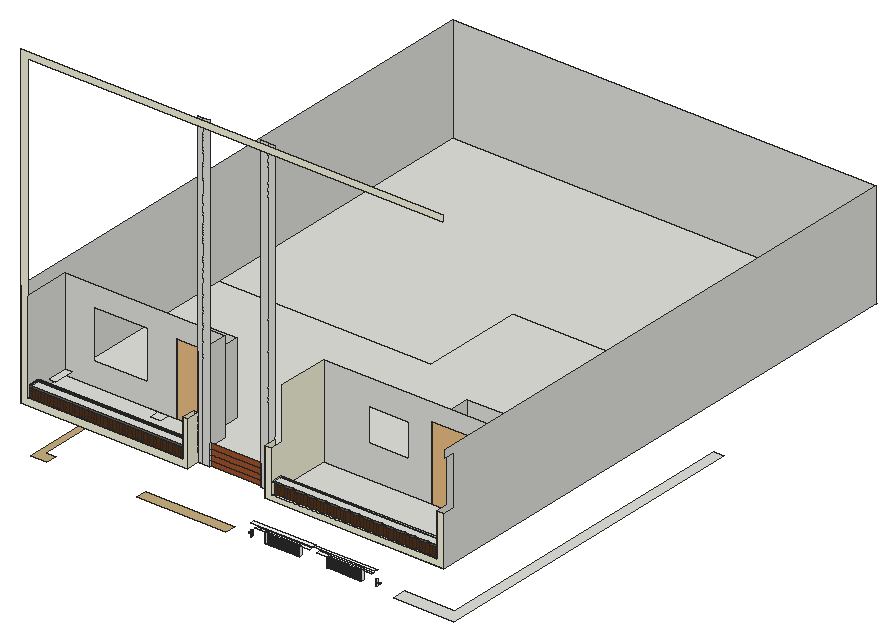
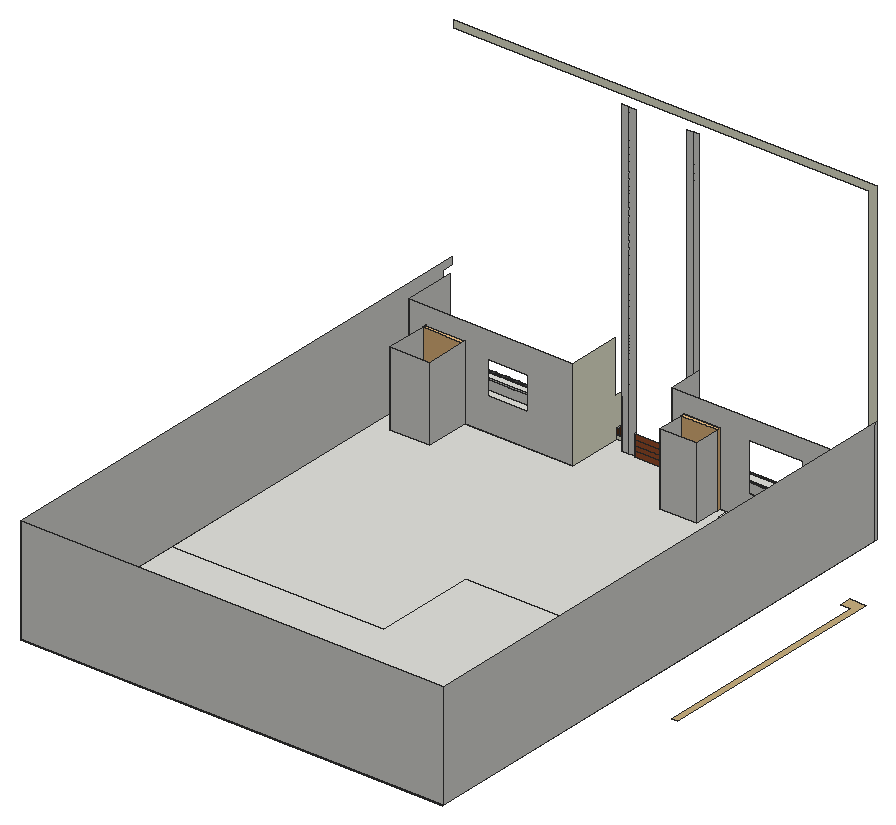
# SketchUp Ruby script. Lengths in inches.
U = 1.inch
M = Sketchup.active_model
def pt(a) = Geom::Point3d.new(a.map { |v| v * U })
def face(e, loops, mat)
  f = e.add_face(loops[0].map { |a| pt(a) })
  loops[1..].each { |l| e.add_face(l.map { |a| pt(a) }).erase! }
  f.material = f.back_material = mat if mat
  f
end
# faces: each face lists its corners as indices into pts; further lists are holes
def faces(e, pts, list, mat = nil) = list.each { |f| face(e, (f[0].is_a?(Array) ? f : [f]).map { |l| l.map { |i| pts[i] } }, mat) }
# xy, xz, yz: faces in a plane at the given z, y or x. An outline is a flat list of corners, or four numbers for a rectangle; further outlines are holes
def ring(l) = l.size == 4 ? [[l[0], l[1]], [l[2], l[1]], [l[2], l[3]], [l[0], l[3]]] : l.each_slice(2).to_a
def flat(e, list, mat, &to3) = list.each { |f| face(e, (f[0].is_a?(Array) ? f : [f]).map { |l| ring(l).map { |u, v| to3.(u, v) } }, mat) }
def xy(e, z, list, mat = nil) = flat(e, list, mat) { |x, y| [x, y, z] }
def xz(e, y, list, mat = nil) = flat(e, list, mat) { |x, z| [x, y, z] }
def yz(e, x, list, mat = nil) = flat(e, list, mat) { |y, z| [x, y, z] }
def lines(e, pts, list) = list.each { |a, b| e.add_line(pt(pts[a]), pt(pts[b])) }
# prism: a flat outline (further loops are holes) pulled along v
def prism(e, loops, v, mat = nil)
  f = face(e, loops, mat); d = Geom::Vector3d.new(v.map { |x| x * U })
  f.pushpull(f.normal.samedirection?(d) ? d.length : -d.length)
end
def box(e, o, s, mat = nil) = prism(e, [[o, [o[0] + s[0], o[1], o[2]], [o[0] + s[0], o[1] + s[1], o[2]], [o[0], o[1] + s[1], o[2]]]], [0, 0, s[2]], mat)
def at(x, y, z, deg = 0) = Geom::Transformation.translation(pt([x, y, z])) * Geom::Transformation.rotation(ORIGIN, Z_AXIS, deg.degrees)
def axes(o, x, y, z) = Geom::Transformation.new([*x, 0, *y, 0, *z, 0, *pt(o).to_a, 1])
def part(name) = M.definitions.add(name)
# library, detail: a bought-in or finely detailed component or shape, given as its bounding box
def library(name, o, s) = part(name).tap { |d| box(d.entities, o, s) }
def detail(e, o, s) = box(e.add_group.entities, o, s)
def put(e, d, t, mat = nil) = e.add_instance(d, t).tap { |i| i.material = mat if mat }
def group(e, t, mat = nil) = e.add_group.tap { |g| g.transformation = t; g.material = mat if mat }.entities
root = M.entities
M.materials.add("[0042_Sienna]").color = [160, 82, 45]
M.materials.add("[0049_Beige]").color = [245, 245, 220]
M.materials.add("[0134_DimGray]").color = [105, 105, 105]
M.materials.add("[Color_000]").color = [255, 255, 255]
M.materials.add("[Color_C20]").color = [102, 91, 81]
M.materials.add("[Roofing Slate Tan]").color = [200, 175, 128]
M.materials.add("[Wood Cherry Original]").color = [86, 49, 23]
c1 = part("Horizontal gate slat")
xy(c1.entities,0,[[0.39,114.16,6.3,114.17]])
xy(c1.entities,0,[[0.39,0,6.3,114.16]],"[Color_C20]")
xy(c1.entities,0.39,[[0.39,0,0.79,114.17],[0.98,0,2.07,114.17],[2.36,0,3.2,114.17],[3.59,0,4.37,114.17],[4.56,0,5.71,114.17],
  [5.91,0,6.3,114.17]],"[Color_C20]")
xy(c1.entities,0.79,[[0.39,0,0.79,114.17],[0.98,0,2.07,114.17],[2.36,0,3.2,114.17],[3.59,0,4.37,114.17],[4.56,0,5.71,114.17],
  [5.91,0,6.3,114.17]],"[Color_C20]")
xy(c1.entities,0.99,[[1.13,0,1.21,114.16],[1.87,0,1.94,114.16],[2.61,0,2.68,114.16],[3.35,0,3.42,114.16],[4.08,0,4.16,114.16],
  [4.82,0,4.9,114.16],[5.5625,0,5.63,114.16],[6.3,0,6.37,114.16]],"[Color_C20]")
xy(c1.entities,1.18,[[0.39,114.16,3.35,114.17],[3.35,114.16,6.3,114.17]])
xy(c1.entities,1.18,[[0.39,0,1.13,114.16],[1.21,0,1.87,114.16],[1.94,0,2.61,114.16],[2.68,0,3.35,114.16],[3.42,0,4.08,114.16],
  [4.16,0,4.82,114.16],[4.9,0,5.5625,114.16],[5.63,0,6.3,114.16]],"[Color_C20]")
xz(c1.entities,0,[[[0.39,0,6.3,0,6.3,0.39,5.91,0.39,5.91,0.79,6.3,0.79,6.3,1.18,5.63,1.18,5.63,0.99,5.5625,0.99,5.5625,1.18,4.9,1.18,4.9,0.99,4.82,0.99,4.82,1.18,4.16,1.18,4.16,0.99,4.08,0.99,4.08,1.18,3.42,1.18,3.42,0.99,3.35,0.99,3.35,1.18,2.68,1.18,2.68,0.99,2.61,0.99,2.61,1.18,1.94,1.18,1.94,0.99,1.87,0.99,1.87,1.18,1.21,1.18,1.21,0.99,1.13,0.99,1.13,1.18,0.39,1.18,0.39,0.79,0.79,0.79,0.79,0.39,0.39,0.39],[4.56,0.39,5.71,0.79],[0.98,0.39,2.07,0.79],[2.36,0.39,3.2,0.79],[3.59,0.39,4.37,0.79]],[6.3,0.99,6.37,1.18]],"[Color_C20]")
xz(c1.entities,114.16,[[1.13,0.99,1.21,1.18],[1.87,0.99,1.94,1.18],[2.61,0.99,2.68,1.18],[3.35,0.99,3.42,1.18],[4.08,0.99,4.16,1.18],
  [4.82,0.99,4.9,1.18],[5.5625,0.99,5.63,1.18]],"[Color_C20]")
xz(c1.entities,114.17,[[[0.39,0,0.39,0.39,0.79,0.39,0.79,0.79,0.39,0.79,0.39,1.18,6.3,1.18,6.3,0.79,5.91,0.79,5.91,0.39,6.3,0.39,6.3,0],[4.56,0.39,5.71,0.79],[0.98,0.39,2.07,0.79],[2.36,0.39,3.2,0.79],[3.59,0.39,4.37,0.79]]],"[Color_C20]")
yz(c1.entities,0.39,[[114.16,0,114.17,0.39],[114.16,0.79,114.17,1.18]])
yz(c1.entities,0.39,[[0,0,114.16,0.39],[0,0.79,114.16,1.18]],"[Color_C20]")
yz(c1.entities,0.79,[[0,0.39,114.17,0.79]],"[Color_C20]")
yz(c1.entities,0.98,[[0,0.39,114.17,0.79]],"[Color_C20]")
yz(c1.entities,1.13,[[0,0.99,114.16,1.18]],"[Color_C20]")
yz(c1.entities,1.21,[[0,0.99,114.16,1.18]],"[Color_C20]")
yz(c1.entities,1.87,[[0,0.99,114.16,1.18]],"[Color_C20]")
yz(c1.entities,1.94,[[0,0.99,114.16,1.18]],"[Color_C20]")
yz(c1.entities,2.07,[[0,0.39,114.17,0.79]],"[Color_C20]")
yz(c1.entities,2.36,[[0,0.39,114.17,0.79]],"[Color_C20]")
yz(c1.entities,2.61,[[0,0.99,114.16,1.18]],"[Color_C20]")
yz(c1.entities,2.68,[[0,0.99,114.16,1.18]],"[Color_C20]")
yz(c1.entities,3.2,[[0,0.39,114.17,0.79]],"[Color_C20]")
yz(c1.entities,3.35,[[0,0.99,114.16,1.18]],"[Color_C20]")
yz(c1.entities,3.42,[[0,0.99,114.16,1.18]],"[Color_C20]")
yz(c1.entities,3.59,[[0,0.39,114.17,0.79]],"[Color_C20]")
yz(c1.entities,4.08,[[0,0.99,114.16,1.18]],"[Color_C20]")
yz(c1.entities,4.16,[[0,0.99,114.16,1.18]],"[Color_C20]")
yz(c1.entities,4.37,[[0,0.39,114.17,0.79]],"[Color_C20]")
yz(c1.entities,4.56,[[0,0.39,114.17,0.79]],"[Color_C20]")
yz(c1.entities,4.82,[[0,0.99,114.16,1.18]],"[Color_C20]")
yz(c1.entities,4.9,[[0,0.99,114.16,1.18]],"[Color_C20]")
yz(c1.entities,5.5625,[[0,0.99,114.16,1.18]],"[Color_C20]")
yz(c1.entities,5.63,[[0,0.99,114.16,1.18]],"[Color_C20]")
yz(c1.entities,5.71,[[0,0.39,114.17,0.79]],"[Color_C20]")
yz(c1.entities,5.91,[[0,0.39,114.17,0.79]],"[Color_C20]")
yz(c1.entities,6.3,[[114.16,0,114.17,0.39],[114.16,0.79,114.17,1.18]])
yz(c1.entities,6.3,[[0,0,114.16,0.39],[0,0.79,114.16,0.99],[0,0.99,114.16,1.18]],"[Color_C20]")
yz(c1.entities,6.37,[[0,0.99,114.16,1.18]],"[Color_C20]")
p = [[0,0,0],[0.39,0,0]]
lines(c1.entities,p,[[0,1]])
c2 = part("Vertical gate panel")
put(c2.entities,c1,axes([0,1.18,0],[3.67755,0,0],[0,0,2.40086],[0,-1,0]))
put(c2.entities,c1,axes([21.72,1.18,0],[3.67755,0,0],[0,0,2.40086],[0,-1,0]))
c3 = library("PINTU 6 YA",[0,-0.6875,0],[35.83,8.07,80.71])
xy(root,60,[[411.91,15.9375,480,15.9375,480,400.0625,468.66,400.0625,468.66,32.24,411.91,32.24]])
xy(root,60,[[0,15.9375,18.32,15.9375,18.32,28.66,6.6875,28.66,6.6875,283.1875,0,283.1875],[120.04,15.9375,221.75,28.66]],"[Roofing Slate Tan]")
xy(root,60.9375,[[263.68,20.54,299.69,24.42],[334.15,20.54,370.17,24.16]],"[Color_000]")
xy(root,61.26,[[387.25,21.82,388.53,23.18],[245.3125,21.91,246.59,23.37]],"[Color_000]")
xy(root,64,[[387.25,21.82,388.53,23.18],[245.3125,21.91,246.59,23.37]],"[Color_000]")
xy(root,64.12,[[387.25,21.82,388.53,23.18],[388.53,21.82,391.17,23.18],[242.68,21.91,245.3125,23.37],[245.3125,21.91,246.59,23.37]],"[Color_000]")
xy(root,64.95,[[387.25,21.82,388.53,23.18],[388.53,21.82,391.17,23.18],[242.68,21.91,245.3125,23.37],[245.3125,21.91,246.59,23.37]],"[Color_000]")
xy(root,65.08,[[387.25,21.82,388.53,23.18],[245.3125,21.91,246.59,23.37]],"[Color_000]")
xy(root,67.71,[[387.25,21.82,388.53,23.18],[245.3125,21.91,246.59,23.37]],"[Color_000]")
xy(root,72.27,[[250.625,20.54,256.29,24.42],[256.29,20.54,261.95,24.42],[263.68,20.54,299.69,24.42],[301.41,20.54,312.74,24.42],[321.1,20.54,332.43,24.16],
  [334.15,20.54,370.17,24.16],[371.89,20.54,377.56,24.16],[377.56,20.54,383.22,24.16]],"[Color_000]")
xy(root,76.3,[[246.59,20.54,316.77,24.42],[317.07,20.54,387.25,24.16]],"[Color_000]")
xy(root,99.91,[[339.53,400.0625,401.28,485.1875]])
xy(root,120,[[0,1,0,283.1875,240,283.1875,240,400.0625,480,400.0625,480,2.0625,276.8125,2.0625,276.8125,15.9375,260.98,15.9375,260.98,17.375,203.35,17.375,203.35,15.9375,189.625,15.9375,189.625,1],[0,283.1875,0,614.8125,480,614.8125,480,400.0625,240,400.0625,240,283.1875],[0,614.8125,480,615.9375]])
xy(root,126.6875,[[284.8125,2.0625,472,4.5]])
xy(root,126.8125,[[77.42,42.13,90.17,67.13]])
xy(root,127.875,[[8,3.0625,185,15.9375]])
xy(root,128,[[8,1,185,2.5625],[8,2.5625,11.54,3.0625],[11.54,2.5625,15.08,3.0625],[15.08,2.5625,18.62,3.0625],[18.62,2.5625,22.16,3.0625],
  [22.16,2.5625,25.7,3.0625],[25.7,2.5625,29.24,3.0625],[29.24,2.5625,32.78,3.0625],[32.78,2.5625,36.32,3.0625],[36.32,2.5625,39.86,3.0625],
  [39.86,2.5625,43.4,3.0625],[43.4,2.5625,46.94,3.0625],[46.94,2.5625,50.48,3.0625],[50.48,2.5625,54.02,3.0625],[54.02,2.5625,57.56,3.0625],
  [57.56,2.5625,61.1,3.0625],[61.1,2.5625,64.64,3.0625],[64.64,2.5625,68.18,3.0625],[68.18,2.5625,71.72,3.0625],[71.72,2.5625,75.26,3.0625],
  [75.26,2.5625,78.8,3.0625],[78.8,2.5625,82.34,3.0625],[82.34,2.5625,85.88,3.0625],[85.88,2.5625,89.42,3.0625],[89.42,2.5625,92.96,3.0625],
  [92.96,2.5625,96.5,3.0625],[96.5,2.5625,100.04,3.0625],[100.04,2.5625,103.58,3.0625],[103.58,2.5625,107.12,3.0625],[107.12,2.5625,110.66,3.0625],
  [110.66,2.5625,114.2,3.0625],[114.2,2.5625,117.74,3.0625],[117.74,2.5625,121.28,3.0625],[121.28,2.5625,124.82,3.0625],[124.82,2.5625,128.36,3.0625],
  [128.36,2.5625,131.9,3.0625],[131.9,2.5625,135.44,3.0625],[135.44,2.5625,138.98,3.0625],[138.98,2.5625,142.52,3.0625],[142.52,2.5625,146.06,3.0625],
  [146.06,2.5625,149.6,3.0625],[149.6,2.5625,153.14,3.0625],[153.14,2.5625,156.68,3.0625],[156.68,2.5625,160.22,3.0625],[160.22,2.5625,163.76,3.0625],
  [163.76,2.5625,167.3,3.0625],[167.3,2.5625,170.84,3.0625],[170.84,2.5625,174.38,3.0625],[174.38,2.5625,177.92,3.0625],[177.92,2.5625,181.46,3.0625],
  [181.46,2.5625,185,3.0625],[[8,3.0625,185,3.0625,185,15.9375,189.625,15.9375,189.625,54.5,175.6875,54.5,175.6875,88.25,134.5,88.25,134.5,54.5,126.45,54.5,126.45,42.13,113.7,42.13,113.7,54.5,8,54.5],[149.98,42.13,162.73,67.13]],[284.8125,14.97,472,14.97,472,75.125,452.27,75.125,452.27,125.625,407.59,125.625,407.59,75.125,284.8125,75.125],[113.7,42.13,126.45,54.5],[113.7,54.5,126.45,67.13]])
xy(root,134.54,[[7.64,30.94,16.14,60.82]])
xy(root,138.5625,[[8,2.5625,185,15.9375],[284.8125,3.0625,472,4.5],[284.8125,4.5,472,14.97]])
xz(root,1,[[0,120,189.625,120,189.625,170.625,185,170.625,185,128,8,128,8,472.625,480,472.625,480,480,0,480]],"[0049_Beige]")
xz(root,2.0625,[[276.8125,120,480,120,480,175.875,472,175.875,472,126.6875,284.8125,126.6875,284.8125,173.625,276.8125,173.625]],"[0049_Beige]")
xz(root,2.5625,[[8,138.5625,185,140.5625]],"[0134_DimGray]")
xz(root,2.5625,[[8,128,11.54,138.5625],[11.54,128,15.08,138.5625],[15.08,128,18.62,138.5625],[18.62,128,22.16,138.5625],[22.16,128,25.7,138.5625],
  [25.7,128,29.24,138.5625],[29.24,128,32.78,138.5625],[32.78,128,36.32,138.5625],[36.32,128,39.86,138.5625],[39.86,128,43.4,138.5625],
  [43.4,128,46.94,138.5625],[46.94,128,50.48,138.5625],[50.48,128,54.02,138.5625],[54.02,128,57.56,138.5625],[57.56,128,61.1,138.5625],
  [61.1,128,64.64,138.5625],[64.64,128,68.18,138.5625],[68.18,128,71.72,138.5625],[71.72,128,75.26,138.5625],[75.26,128,78.8,138.5625],
  [78.8,128,82.34,138.5625],[82.34,128,85.88,138.5625],[85.88,128,89.42,138.5625],[89.42,128,92.96,138.5625],[92.96,128,96.5,138.5625],
  [96.5,128,100.04,138.5625],[100.04,128,103.58,138.5625],[103.58,128,107.12,138.5625],[107.12,128,110.66,138.5625],[110.66,128,114.2,138.5625],
  [114.2,128,117.74,138.5625],[117.74,128,121.28,138.5625],[121.28,128,124.82,138.5625],[124.82,128,128.36,138.5625],[128.36,128,131.9,138.5625],
  [131.9,128,135.44,138.5625],[135.44,128,138.98,138.5625],[138.98,128,142.52,138.5625],[142.52,128,146.06,138.5625],[146.06,128,149.6,138.5625],
  [149.6,128,153.14,138.5625],[153.14,128,156.68,138.5625],[156.68,128,160.22,138.5625],[160.22,128,163.76,138.5625],[163.76,128,167.3,138.5625],
  [167.3,128,170.84,138.5625],[170.84,128,174.38,138.5625],[174.38,128,177.92,138.5625],[177.92,128,181.46,138.5625],[181.46,128,185,138.5625]],"[Wood Cherry Original]")
xz(root,3.0625,[[8,127.875,185,128]])
xz(root,3.0625,[[284.8125,138.5625,292.3,140.3125],[292.3,138.5625,296.04,140.3125],[296.04,138.5625,299.79,140.3125],[299.79,138.5625,303.53,140.3125],[303.53,138.5625,307.28,140.3125],
  [307.28,138.5625,311.02,140.3125],[311.02,138.5625,314.76,140.3125],[314.76,138.5625,318.51,140.3125],[318.51,138.5625,322.25,140.3125],[322.25,138.5625,325.99,140.3125],
  [325.99,138.5625,329.74,140.3125],[329.74,138.5625,333.48,140.3125],[333.48,138.5625,337.22,140.3125],[337.22,138.5625,340.97,140.3125],[340.97,138.5625,344.71,140.3125],
  [344.71,138.5625,348.46,140.3125],[348.46,138.5625,352.2,140.3125],[352.2,138.5625,355.94,140.3125],[355.94,138.5625,359.6875,140.3125],[359.6875,138.5625,363.43,140.3125],
  [363.43,138.5625,367.17,140.3125],[367.17,138.5625,370.92,140.3125],[370.92,138.5625,374.66,140.3125],[374.66,138.5625,378.41,140.3125],[378.41,138.5625,382.15,140.3125],
  [382.15,138.5625,385.89,140.3125],[385.89,138.5625,389.64,140.3125],[389.64,138.5625,393.38,140.3125],[393.38,138.5625,397.125,140.3125],[397.125,138.5625,400.87,140.3125],
  [400.87,138.5625,404.61,140.3125],[404.61,138.5625,408.36,140.3125],[408.36,138.5625,412.1,140.3125],[412.1,138.5625,415.84,140.3125],[415.84,138.5625,419.59,140.3125],
  [419.59,138.5625,423.33,140.3125],[423.33,138.5625,427.08,140.3125],[427.08,138.5625,430.82,140.3125],[430.82,138.5625,434.5625,140.3125],[434.5625,138.5625,438.31,140.3125],
  [438.31,138.5625,442.05,140.3125],[442.05,138.5625,445.79,140.3125],[445.79,138.5625,449.54,140.3125],[449.54,138.5625,453.28,140.3125],[453.28,138.5625,457.03,140.3125],
  [457.03,138.5625,460.77,140.3125],[460.77,138.5625,464.51,140.3125],[464.51,138.5625,468.26,140.3125],[468.26,138.5625,472,140.3125]],"[0134_DimGray]")
xz(root,4.5,[[284.8125,126.6875,288.56,138.5625],[288.56,126.6875,292.3,138.5625],[292.3,126.6875,296.04,138.5625],[296.04,126.6875,299.79,138.5625],[299.79,126.6875,303.53,138.5625],
  [303.53,126.6875,307.28,138.5625],[307.28,126.6875,311.02,138.5625],[311.02,126.6875,314.76,138.5625],[314.76,126.6875,318.51,138.5625],[318.51,126.6875,322.25,138.5625],
  [322.25,126.6875,325.99,138.5625],[325.99,126.6875,329.74,138.5625],[329.74,126.6875,333.48,138.5625],[333.48,126.6875,337.22,138.5625],[337.22,126.6875,340.97,138.5625],
  [340.97,126.6875,344.71,138.5625],[344.71,126.6875,348.46,138.5625],[348.46,126.6875,352.2,138.5625],[352.2,126.6875,355.94,138.5625],[355.94,126.6875,359.6875,138.5625],
  [359.6875,126.6875,363.43,138.5625],[363.43,126.6875,367.17,138.5625],[367.17,126.6875,370.92,138.5625],[370.92,126.6875,374.66,138.5625],[374.66,126.6875,378.41,138.5625],
  [378.41,126.6875,382.15,138.5625],[382.15,126.6875,385.89,138.5625],[385.89,126.6875,389.64,138.5625],[389.64,126.6875,393.38,138.5625],[393.38,126.6875,397.125,138.5625],
  [397.125,126.6875,400.87,138.5625],[400.87,126.6875,404.61,138.5625],[404.61,126.6875,408.36,138.5625],[408.36,126.6875,412.1,138.5625],[412.1,126.6875,415.84,138.5625],
  [415.84,126.6875,419.59,138.5625],[419.59,126.6875,423.33,138.5625],[423.33,126.6875,427.08,138.5625],[427.08,126.6875,430.82,138.5625],[430.82,126.6875,434.5625,138.5625],
  [434.5625,126.6875,438.31,138.5625],[438.31,126.6875,442.05,138.5625],[442.05,126.6875,445.79,138.5625],[445.79,126.6875,449.54,138.5625],[449.54,126.6875,453.28,138.5625],
  [453.28,126.6875,457.03,138.5625],[457.03,126.6875,460.77,138.5625],[460.77,126.6875,464.51,138.5625],[464.51,126.6875,468.26,138.5625],[468.26,126.6875,472,138.5625]],"[Wood Cherry Original]")
xz(root,14.97,[[284.8125,128,472,138.5625],[284.8125,138.5625,472,140.3125]])
xz(root,15.9375,[[189.625,120,195.35,120,195.35,472.625,189.625,472.625,189.625,374,190.03,374,190.03,372,189.625,372,189.625,360,190.03,360,190.03,352,189.625,352,189.625,252.875,190.625,252.875,190.625,251.875,189.625,251.875,189.625,173.625,190.625,173.625,190.625,170.625,189.625,170.625],[195.35,120,203.35,472.625],[260.98,120,268.98,472.625],[268.98,120,276.8125,120,276.8125,173.625,275.8125,173.625,275.8125,175.875,276.8125,175.875,276.8125,472.625,268.98,472.625],[8,127.875,185,138.5625],
  [185,128,189.625,170.625],[8,138.5625,185,139.5625],[8,139.5625,185,140.5625]])
xz(root,17.375,[[203.35,120,260.98,125.88],[203.35,125.88,260.98,131.75],[203.35,131.75,260.98,137.63],[203.35,137.63,260.98,143.51]],"[0042_Sienna]")
xz(root,20.54,[[261.95,60.9375,263.68,72.27],[299.69,60.9375,301.41,72.27],[332.43,60.9375,334.15,72.27],[370.17,60.9375,371.89,72.27]],"[Color_000]")
xz(root,21.82,[[387.25,61.26,388.53,64],[387.25,64.12,391.17,64.95],[387.25,65.08,388.53,67.71]],"[Color_000]")
xz(root,21.91,[[245.3125,61.26,246.59,64],[242.68,64.12,246.59,64.95],[245.3125,65.08,246.59,67.71]],"[Color_000]")
xz(root,23.18,[[387.25,61.26,388.53,64],[387.25,64.12,388.53,64.44],[388.53,64.12,388.53,64.44,387.25,64.44,387.25,64.95,391.17,64.95,391.17,64.12],[387.25,65.08,388.53,67.71]],"[Color_000]")
xz(root,23.37,[[245.3125,61.26,246.59,64],[242.68,64.12,242.68,64.95,246.59,64.95,246.59,64.44,245.3125,64.44,245.3125,64.12],[245.3125,64.12,246.59,64.44],[245.3125,65.08,246.59,67.71]],"[Color_000]")
xz(root,54.5,[[[8,128,134.5,128,134.5,209.5,175.6875,209.5,175.6875,128,189.625,128,189.625,231.875,8,231.875],[41.11,154.08,102.36,209.33]]])
xz(root,75.125,[[[284.8125,128,407.59,128,407.59,211.875,452.27,211.875,452.27,128,472,128,472,231.875,284.8125,231.875],[336.13,165.23,382.38,202.54]]])
xz(root,88.25,[[134.5,128,175.6875,209.5]])
xz(root,125.625,[[407.59,128,452.27,211.875]])
xz(root,614.8125,[[0,120,480,239.875]])
yz(root,0,[[1,120,3.0625,239.875],[3.0625,120,614.8125,239.875]])
yz(root,8,[[3.0625,127.875,15.9375,128],[1,128,2.5625,128,2.5625,140.5625,15.9375,140.5625,15.9375,128,54.5,128,54.5,231.875,1,231.875],[2.5625,128,15.9375,138.5625],[2.5625,138.5625,15.9375,139.5625],[2.5625,139.5625,15.9375,140.5625]])
yz(root,134.5,[[54.5,128,88.25,209.5]])
yz(root,175.6875,[[54.5,128,88.25,209.5]])
yz(root,185,[[3.0625,127.875,15.9375,128],[2.5625,128,15.9375,138.5625],[2.5625,138.5625,15.9375,139.5625],[2.5625,139.5625,15.9375,140.5625]])
yz(root,185,[[1,128,1,170.625,15.9375,170.625,15.9375,140.5625,2.5625,140.5625,2.5625,128]],"[0049_Beige]")
yz(root,189.625,[[15.9375,128,54.5,231.875]])
yz(root,189.625,[[1,120,15.9375,170.625]],"[0049_Beige]")
yz(root,203.35,[[15.9375,120,17.375,125.88],[15.9375,125.88,17.375,131.75],[15.9375,131.75,17.375,137.63],[15.9375,137.63,17.375,143.51]])
yz(root,242.68,[[21.91,64.12,23.37,64.95]],"[Color_000]")
yz(root,245.3125,[[21.91,61.26,23.37,64],[21.91,65.08,23.37,67.71]],"[Color_000]")
yz(root,260.98,[[15.9375,120,17.375,125.88],[15.9375,125.88,17.375,131.75],[15.9375,131.75,17.375,137.63],[15.9375,137.63,17.375,143.51]])
yz(root,261.95,[[20.54,60.9375,24.42,72.27]],"[Color_000]")
yz(root,263.68,[[20.54,60.9375,24.42,72.27]],"[Color_000]")
yz(root,276.8125,[[2.0625,120,15.9375,173.625]],"[0049_Beige]")
yz(root,284.8125,[[3.0625,138.5625,14.97,140.3125]])
yz(root,284.8125,[[2.0625,126.6875,4.5,126.6875,4.5,138.5625,3.0625,138.5625,3.0625,140.3125,14.97,140.3125,14.97,128,75.125,128,75.125,231.875,15.9375,231.875,15.9375,173.625,2.0625,173.625]],"[0049_Beige]")
yz(root,299.69,[[20.54,60.9375,24.42,72.27]],"[Color_000]")
yz(root,301.41,[[20.54,60.9375,24.42,72.27]],"[Color_000]")
yz(root,332.43,[[20.54,60.9375,24.16,72.27]],"[Color_000]")
yz(root,334.15,[[20.54,60.9375,24.16,72.27]],"[Color_000]")
yz(root,370.17,[[20.54,60.9375,24.16,72.27]],"[Color_000]")
yz(root,371.89,[[20.54,60.9375,24.16,72.27]],"[Color_000]")
yz(root,388.53,[[21.82,61.26,23.18,64],[21.82,65.08,23.18,67.71]],"[Color_000]")
yz(root,407.59,[[75.125,128,125.625,211.875]])
yz(root,452.27,[[75.125,128,125.625,211.875]])
yz(root,472,[[2.0625,126.6875,2.0625,175.875,15.9375,175.875,15.9375,231.875,75.125,231.875,75.125,128,14.97,128,14.97,140.3125,3.0625,140.3125,3.0625,138.5625,4.5,138.5625,4.5,126.6875],[3.0625,138.5625,14.97,140.3125]])
yz(root,480,[[2.0625,120,614.8125,120,614.8125,239.875,3.0625,239.875,3.0625,231.875,15.9375,231.875,15.9375,175.875,2.0625,175.875]])
p = [[375.45,21.14,72.26],[334.15,21.14,72.26],[258.39,21.1875,72.26],[299.69,21.1875,72.26],[246.59,23.37,64.12],[246.59,23.37,64]]
lines(root,p,[[0,1],[2,3],[4,5]])
put(root,c2,axes([334.15,21.14,60.25],[0,0,0.2676],[0,0.24487,0],[0.13139,0,0]))
put(root,c2,axes([299.69,21.1875,60.25],[0,0,0.2676],[0,0.2624,0],[-0.13139,0,0]))
put(root,c3,axes([134.5,54.82,128],[1.14953,0,0],[0,0.45732,0],[0,0,1.01677]),"[0042_Sienna]")
put(root,c3,axes([407.96,75.125,128],[1.23668,0,0],[0,0.5,0],[0,0,1.03923]))
